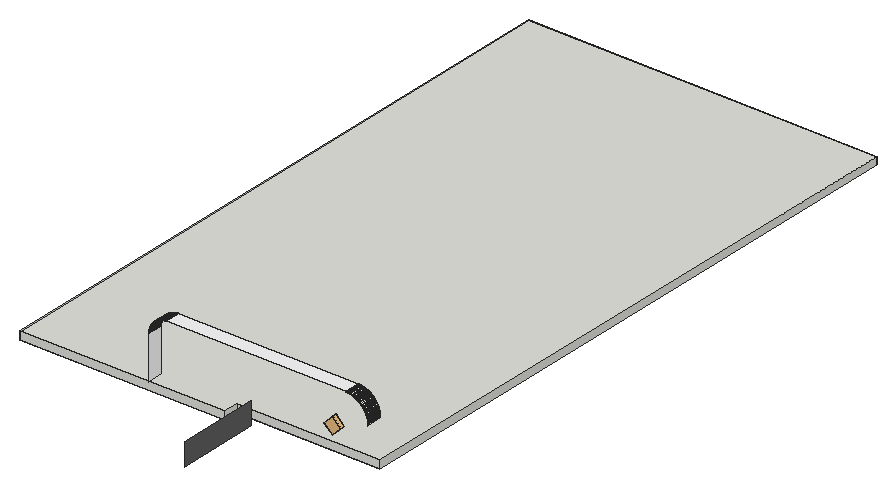
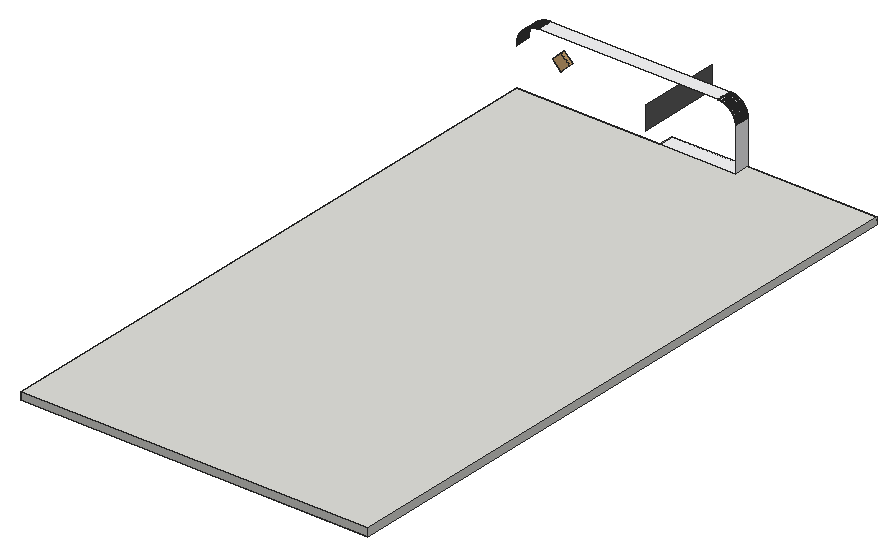
# SketchUp Ruby script. Lengths in inches.
U = 1.inch
M = Sketchup.active_model
def pt(a) = Geom::Point3d.new(a.map { |v| v * U })
def face(e, loops, mat)
  f = e.add_face(loops[0].map { |a| pt(a) })
  loops[1..].each { |l| e.add_face(l.map { |a| pt(a) }).erase! }
  f.material = f.back_material = mat if mat
  f
end
# faces: each face lists its corners as indices into pts; further lists are holes
def faces(e, pts, list, mat = nil) = list.each { |f| face(e, (f[0].is_a?(Array) ? f : [f]).map { |l| l.map { |i| pts[i] } }, mat) }
# xy, xz, yz: faces in a plane at the given z, y or x. An outline is a flat list of corners, or four numbers for a rectangle; further outlines are holes
def ring(l) = l.size == 4 ? [[l[0], l[1]], [l[2], l[1]], [l[2], l[3]], [l[0], l[3]]] : l.each_slice(2).to_a
def flat(e, list, mat, &to3) = list.each { |f| face(e, (f[0].is_a?(Array) ? f : [f]).map { |l| ring(l).map { |u, v| to3.(u, v) } }, mat) }
def xy(e, z, list, mat = nil) = flat(e, list, mat) { |x, y| [x, y, z] }
def xz(e, y, list, mat = nil) = flat(e, list, mat) { |x, z| [x, y, z] }
def yz(e, x, list, mat = nil) = flat(e, list, mat) { |y, z| [x, y, z] }
def lines(e, pts, list) = list.each { |a, b| e.add_line(pt(pts[a]), pt(pts[b])) }
# prism: a flat outline (further loops are holes) pulled along v
def prism(e, loops, v, mat = nil)
  f = face(e, loops, mat); d = Geom::Vector3d.new(v.map { |x| x * U })
  f.pushpull(f.normal.samedirection?(d) ? d.length : -d.length)
end
def box(e, o, s, mat = nil) = prism(e, [[o, [o[0] + s[0], o[1], o[2]], [o[0] + s[0], o[1] + s[1], o[2]], [o[0], o[1] + s[1], o[2]]]], [0, 0, s[2]], mat)
def at(x, y, z, deg = 0) = Geom::Transformation.translation(pt([x, y, z])) * Geom::Transformation.rotation(ORIGIN, Z_AXIS, deg.degrees)
def axes(o, x, y, z) = Geom::Transformation.new([*x, 0, *y, 0, *z, 0, *pt(o).to_a, 1])
def part(name) = M.definitions.add(name)
# library, detail: a bought-in or finely detailed component or shape, given as its bounding box
def library(name, o, s) = part(name).tap { |d| box(d.entities, o, s) }
def detail(e, o, s) = box(e.add_group.entities, o, s)
def put(e, d, t, mat = nil) = e.add_instance(d, t).tap { |i| i.material = mat if mat }
def group(e, t, mat = nil) = e.add_group.tap { |g| g.transformation = t; g.material = mat if mat }.entities
root = M.entities
M.materials.add("1421 AP 8232 ELEGANT GREY").color = [96, 96, 96]
M.materials.add("1448 AP 8253 RAVEN SONG").color = [0, 0, 0]
M.materials.add("[Quartz Light Grey]").color = [251, 251, 252]
c1 = library("Group\#22",[-1.75,-3,-1.85],[9.46,3.28,9.45])
xy(root,246,[[[36,271,198,271,198,283,312,283,312,775,36,775],[45,280,45,766,303,766,303,292,189,292,189,280]]])
xy(root,252,[[138,271,198,283]],"[Quartz Light Grey]")
xy(root,299.99,[[294.47,271,294.71,283]],"[Quartz Light Grey]")
xy(root,300,[[151.63,271,151.82,283],[151.82,271,152,283],[152,271,294,283],[294,271,294.24,283]],"[Quartz Light Grey]")
yz(root,138,[[271,252,283,286],[271,286,283,286.18],[271,286.18,283,286.37]],"[Quartz Light Grey]")
yz(root,219,[[205,249,271,267]],"1421 AP 8232 ELEGANT GREY")
yz(root,311.99,[[271,282.47,283,282.71]],"[Quartz Light Grey]")
yz(root,312,[[271,282,283,282.24]],"[Quartz Light Grey]")
p = [[311.99,271,282.47],[312,271,282.24],[312,283,282.24],[311.99,283,282.47],[311.98,271,282.94],[311.99,271,282.71],
  [311.99,283,282.71],[311.98,283,282.94],[311.96,271,283.18],[311.96,283,283.18],[311.94,271,283.41],[311.94,283,283.41],
  [311.92,271,283.65],[311.92,283,283.65],[311.9,271,283.88],[311.9,283,283.88],[311.875,271,284.12],[311.875,283,284.12],
  [311.85,271,284.35],[311.85,283,284.35],[311.8125,271,284.58],[311.8125,283,284.58],[311.78,271,284.82],[311.78,283,284.82],
  [311.74,271,285.05],[311.74,283,285.05],[311.7,271,285.28],[311.7,283,285.28],[311.65,271,285.51],[311.65,283,285.51],
  [311.61,271,285.74],[311.61,283,285.74],[311.56,271,285.97],[311.56,283,285.97],[311.5,271,286.2],[311.5,283,286.2],
  [311.45,271,286.43],[311.45,283,286.43],[138,271,286.37],[138.01,271,286.55],[138.01,283,286.55],[138,283,286.37],
  [311.39,271,286.66],[311.39,283,286.66],[138.02,271,286.73],[138.02,283,286.73],[138.03,271,286.92],[138.03,283,286.92],
  [311.32,271,286.89],[311.32,283,286.89],[138.04,271,287.1],[138.04,283,287.1],[311.26,271,287.11],[311.26,283,287.11],
  [138.06,271,287.28],[138.06,283,287.28],[311.19,271,287.34],[311.19,283,287.34],[138.08,271,287.46],[138.08,283,287.46],
  [311.12,271,287.5625],[311.12,283,287.5625],[138.1,271,287.65],[138.1,283,287.65],[138.12,271,287.83],[138.12,283,287.83],
  [311.04,271,287.79],[311.04,283,287.79],[138.14,271,288.01],[138.14,283,288.01],[310.97,271,288.01],[310.97,283,288.01],
  [138.17,271,288.19],[138.17,283,288.19],[310.89,271,288.23],[310.89,283,288.23],[138.2,271,288.37],[138.2,283,288.37],
  [310.8,271,288.45],[310.8,283,288.45],[138.23,271,288.55],[138.23,283,288.55],[310.72,271,288.67],[310.72,283,288.67],
  [138.27,271,288.73],[138.27,283,288.73],[138.31,271,288.91],[138.31,283,288.91],[310.63,271,288.89],[310.63,283,288.89],
  [138.35,271,289.09],[138.35,283,289.09],[310.54,271,289.11],[310.54,283,289.11],[138.39,271,289.27],[138.39,283,289.27],
  [310.44,271,289.32],[310.44,283,289.32],[138.43,271,289.45],[138.43,283,289.45],[310.35,271,289.54],[310.35,283,289.54],
  [138.48,271,289.625],[138.48,283,289.625],[310.25,271,289.75],[310.25,283,289.75],[138.53,271,289.8],[138.53,283,289.8],
  [310.14,271,289.96],[310.14,283,289.96],[138.58,271,289.98],[138.58,283,289.98],[138.63,271,290.15],[138.63,283,290.15],
  [310.04,271,290.17],[310.04,283,290.17],[138.69,271,290.33],[138.69,283,290.33],[309.93,271,290.38],[309.93,283,290.38],
  [138.74,271,290.5],[138.74,283,290.5],[309.82,271,290.59],[309.82,283,290.59],[138.8,271,290.67],[138.8,283,290.67],
  [309.7,271,290.8],[309.7,283,290.8],[138.87,271,290.85],[138.87,283,290.85],[138.93,271,291.02],[138.93,283,291.02],
  [309.59,271,291],[309.59,283,291],[139,271,291.1875],[139,283,291.1875],[309.47,271,291.2],[309.47,283,291.2],
  [139.07,271,291.36],[139.07,283,291.36],[309.35,271,291.4],[309.35,283,291.4],[139.14,271,291.53],[139.14,283,291.53],
  [309.22,271,291.61],[309.22,283,291.61],[139.21,271,291.69],[139.21,283,291.69],[309.1,271,291.8],[309.1,283,291.8],
  [139.29,271,291.86],[139.29,283,291.86],[308.97,271,292],[308.97,283,292],[139.36,271,292.03],[139.36,283,292.03],
  [139.44,271,292.19],[139.44,283,292.19],[308.83,271,292.2],[308.83,283,292.2],[139.53,271,292.36],[139.53,283,292.36],
  [308.7,271,292.39],[308.7,283,292.39],[139.61,271,292.52],[139.61,283,292.52],[308.5625,271,292.58],[308.5625,283,292.58],
  [139.7,271,292.68],[139.7,283,292.68],[308.42,271,292.77],[308.42,283,292.77],[139.79,271,292.84],[139.79,283,292.84],
  [139.875,271,293],[139.875,283,293],[308.28,271,292.96],[308.28,283,292.96],[139.97,271,293.16],[139.97,283,293.16],
  [308.14,271,293.14],[308.14,283,293.14],[307.99,271,293.33],[307.99,283,293.33],[140.0625,271,293.31],[140.0625,283,293.31],
  [140.16,271,293.47],[140.16,283,293.47],[307.84,271,293.51],[307.84,283,293.51],[140.26,271,293.625],[140.26,283,293.625],
  [307.6875,271,293.69],[307.6875,283,293.69],[140.36,271,293.78],[140.36,283,293.78],[307.53,271,293.87],[307.53,283,293.87],
  [140.46,271,293.93],[140.46,283,293.93],[140.57,271,294.08],[140.57,283,294.08],[307.375,271,294.04],[307.375,283,294.04],
  [307.22,271,294.22],[307.22,283,294.22],[140.67,271,294.23],[140.67,283,294.23],[140.78,271,294.375],[140.78,283,294.375],
  [307.06,271,294.39],[307.06,283,294.39],[140.89,271,294.52],[140.89,283,294.52],[306.89,271,294.56],[306.89,283,294.56],
  [141.01,271,294.67],[141.01,283,294.67],[306.73,271,294.73],[306.73,283,294.73],[141.12,271,294.81],[141.12,283,294.81],
  [306.56,271,294.89],[306.56,283,294.89],[141.24,271,294.95],[141.24,283,294.95],[306.39,271,295.06],[306.39,283,295.06],
  [141.35,271,295.09],[141.35,283,295.09],[141.47,271,295.23],[141.47,283,295.23],[306.22,271,295.22],[306.22,283,295.22],
  [141.6,271,295.37],[141.6,283,295.37],[306.04,271,295.375],[306.04,283,295.375],[141.72,271,295.5],[141.72,283,295.5],
  [305.87,271,295.53],[305.87,283,295.53],[141.84,271,295.64],[141.84,283,295.64],[305.69,271,295.6875],[305.69,283,295.6875],
  [141.97,271,295.77],[141.97,283,295.77],[305.51,271,295.84],[305.51,283,295.84],[142.1,271,295.9],[142.1,283,295.9],
  [305.33,271,295.99],[305.33,283,295.99],[142.23,271,296.03],[142.23,283,296.03],[142.36,271,296.16],[142.36,283,296.16],
  [305.14,271,296.14],[305.14,283,296.14],[304.96,271,296.28],[304.96,283,296.28],[142.5,271,296.28],[142.5,283,296.28],
  [142.63,271,296.4],[142.63,283,296.4],[304.77,271,296.42],[304.77,283,296.42],[142.77,271,296.53],[142.77,283,296.53],
  [304.58,271,296.5625],[304.58,283,296.5625],[142.91,271,296.65],[142.91,283,296.65],[143.05,271,296.76],[143.05,283,296.76],
  [304.39,271,296.7],[304.39,283,296.7],[304.2,271,296.83],[304.2,283,296.83],[143.19,271,296.88],[143.19,283,296.88],
  [304,271,296.97],[304,283,296.97],[143.33,271,296.99],[143.33,283,296.99],[143.48,271,297.11],[143.48,283,297.11],
  [303.8,271,297.1],[303.8,283,297.1],[143.625,271,297.22],[143.625,283,297.22],[303.61,271,297.22],[303.61,283,297.22],
  [143.77,271,297.33],[143.77,283,297.33],[303.4,271,297.35],[303.4,283,297.35],[143.92,271,297.43],[143.92,283,297.43],
  [303.2,271,297.47],[303.2,283,297.47],[144.07,271,297.54],[144.07,283,297.54],[144.22,271,297.64],[144.22,283,297.64],
  [303,271,297.59],[303,283,297.59],[144.375,271,297.74],[144.375,283,297.74],[302.8,271,297.7],[302.8,283,297.7],
  [144.53,271,297.84],[144.53,283,297.84],[302.59,271,297.82],[302.59,283,297.82],[144.69,271,297.9375],[144.69,283,297.9375],
  [302.38,271,297.93],[302.38,283,297.93],[144.84,271,298.03],[144.84,283,298.03],[302.17,271,298.04],[302.17,283,298.04],
  [145,271,298.125],[145,283,298.125],[301.96,271,298.14],[301.96,283,298.14],[145.16,271,298.21],[145.16,283,298.21],
  [301.75,271,298.25],[301.75,283,298.25],[145.32,271,298.3],[145.32,283,298.3],[301.54,271,298.35],[301.54,283,298.35],
  [145.48,271,298.39],[145.48,283,298.39],[301.32,271,298.44],[301.32,283,298.44],[145.64,271,298.47],[145.64,283,298.47],
  [301.11,271,298.54],[301.11,283,298.54],[145.81,271,298.56],[145.81,283,298.56],[300.89,271,298.63],[300.89,283,298.63],
  [145.97,271,298.64],[145.97,283,298.64],[146.14,271,298.71],[146.14,283,298.71],[300.67,271,298.72],[300.67,283,298.72],
  [146.31,271,298.79],[146.31,283,298.79],[300.45,271,298.8],[300.45,283,298.8],[146.47,271,298.86],[146.47,283,298.86],
  [300.23,271,298.89],[300.23,283,298.89],[146.64,271,298.93],[146.64,283,298.93],[146.8125,271,299],[146.8125,283,299],
  [300.01,271,298.97],[300.01,283,298.97],[146.98,271,299.07],[146.98,283,299.07],[299.5625,271,299.12],[299.79,271,299.04],
  [299.79,283,299.04],[299.5625,283,299.12],[147.15,271,299.13],[147.15,283,299.13],[147.33,271,299.2],[147.33,283,299.2],
  [299.34,271,299.19],[299.34,283,299.19],[147.5,271,299.26],[147.5,283,299.26],[299.11,271,299.26],[299.11,283,299.26],
  [147.67,271,299.31],[147.67,283,299.31],[147.85,271,299.37],[147.85,283,299.37],[298.66,271,299.39],[298.89,271,299.32],
  [298.89,283,299.32],[298.66,283,299.39],[148.02,271,299.42],[148.02,283,299.42],[148.2,271,299.47],[148.2,283,299.47],
  [298.2,271,299.5],[298.43,271,299.45],[298.43,283,299.45],[298.2,283,299.5],[148.375,271,299.52],[148.375,283,299.52],
  [148.55,271,299.57],[148.55,283,299.57],[297.97,271,299.56],[297.97,283,299.56],[148.73,271,299.61],[148.73,283,299.61],
  [148.91,271,299.65],[148.91,283,299.65],[297.51,271,299.65],[297.74,271,299.61],[297.74,283,299.61],[297.51,283,299.65],
  [149.09,271,299.69],[149.09,283,299.69],[149.27,271,299.73],[149.27,283,299.73],[149.45,271,299.77],[149.45,283,299.77],
  [296.82,271,299.78],[297.05,271,299.74],[297.05,283,299.74],[296.82,283,299.78],[297.28,271,299.7],[297.28,283,299.7],
  [149.63,271,299.8],[149.63,283,299.8],[149.81,271,299.83],[149.81,283,299.83],[149.99,271,299.86],[149.99,283,299.86],
  [296.12,271,299.875],[296.35,271,299.85],[296.35,283,299.85],[296.12,283,299.875],[296.58,271,299.8125],[296.58,283,299.8125],
  [150.17,271,299.88],[150.17,283,299.88],[150.35,271,299.9],[150.35,283,299.9],[150.54,271,299.92],[150.54,283,299.92],
  [150.72,271,299.94],[150.72,283,299.94],[150.9,271,299.96],[150.9,283,299.96],[295.18,271,299.96],[295.41,271,299.94],
  [295.41,283,299.94],[295.18,283,299.96],[295.65,271,299.92],[295.65,283,299.92],[295.88,271,299.9],[295.88,283,299.9],
  [151.08,271,299.97],[151.08,283,299.97],[151.27,271,299.98],[151.27,283,299.98],[151.45,271,299.99],[151.45,283,299.99],
  [151.63,271,300],[151.63,283,300],[294.24,271,300],[294.47,271,299.99],[294.47,283,299.99],[294.24,283,300],
  [294.71,271,299.99],[294.94,271,299.98],[294.94,283,299.98],[294.71,283,299.99]]
faces(root,p,[[0,1,2,3],[4,5,6,7],[8,4,7,9],[10,8,9,11],[12,10,11,13],[14,12,13,15],[16,14,15,17],[18,16,17,19],
  [20,18,19,21],[22,20,21,23],[24,22,23,25],[26,24,25,27],[28,26,27,29],[30,28,29,31],[32,30,31,33],[34,32,33,35],
  [36,34,35,37],[38,39,40,41],[42,36,37,43],[39,44,45,40],[44,46,47,45],[48,42,43,49],[46,50,51,47],[52,48,49,53],
  [50,54,55,51],[56,52,53,57],[54,58,59,55],[60,56,57,61],[58,62,63,59],[62,64,65,63],[66,60,61,67],[64,68,69,65],
  [70,66,67,71],[68,72,73,69],[74,70,71,75],[72,76,77,73],[78,74,75,79],[76,80,81,77],[82,78,79,83],[80,84,85,81],
  [84,86,87,85],[88,82,83,89],[86,90,91,87],[92,88,89,93],[90,94,95,91],[96,92,93,97],[94,98,99,95],[100,96,97,101],
  [98,102,103,99],[104,100,101,105],[102,106,107,103],[108,104,105,109],[106,110,111,107],[110,112,113,111],[114,108,109,115],[112,116,117,113],
  [118,114,115,119],[116,120,121,117],[122,118,119,123],[120,124,125,121],[126,122,123,127],[124,128,129,125],[128,130,131,129],[132,126,127,133],
  [130,134,135,131],[136,132,133,137],[134,138,139,135],[140,136,137,141],[138,142,143,139],[144,140,141,145],[142,146,147,143],[148,144,145,149],
  [146,150,151,147],[152,148,149,153],[150,154,155,151],[154,156,157,155],[158,152,153,159],[156,160,161,157],[162,158,159,163],[160,164,165,161],
  [166,162,163,167],[164,168,169,165],[170,166,167,171],[168,172,173,169],[172,174,175,173],[176,170,171,177],[174,178,179,175],[180,176,177,181],
  [182,180,181,183],[178,184,185,179],[184,186,187,185],[188,182,183,189],[186,190,191,187],[192,188,189,193],[190,194,195,191],[196,192,193,197],
  [194,198,199,195],[198,200,201,199],[202,196,197,203],[204,202,203,205],[200,206,207,201],[206,208,209,207],[210,204,205,211],[208,212,213,209],
  [214,210,211,215],[212,216,217,213],[218,214,215,219],[216,220,221,217],[222,218,219,223],[220,224,225,221],[226,222,223,227],[224,228,229,225],
  [228,230,231,229],[232,226,227,233],[230,234,235,231],[236,232,233,237],[234,238,239,235],[240,236,237,241],[238,242,243,239],[244,240,241,245],
  [242,246,247,243],[248,244,245,249],[246,250,251,247],[252,248,249,253],[250,254,255,251],[254,256,257,255],[258,252,253,259],[260,258,259,261],
  [256,262,263,257],[262,264,265,263],[266,260,261,267],[264,268,269,265],[270,266,267,271],[268,272,273,269],[272,274,275,273],[276,270,271,277],
  [278,276,277,279],[274,280,281,275],[282,278,279,283],[280,284,285,281],[284,286,287,285],[288,282,283,289],[286,290,291,287],[292,288,289,293],
  [290,294,295,291],[296,292,293,297],[294,298,299,295],[300,296,297,301],[298,302,303,299],[302,304,305,303],[306,300,301,307],[304,308,309,305],
  [310,306,307,311],[308,312,313,309],[314,310,311,315],[312,316,317,313],[318,314,315,319],[316,320,321,317],[322,318,319,323],[320,324,325,321],
  [326,322,323,327],[324,328,329,325],[330,326,327,331],[328,332,333,329],[334,330,331,335],[332,336,337,333],[338,334,335,339],[336,340,341,337],
  [342,338,339,343],[340,344,345,341],[346,342,343,347],[344,348,349,345],[348,350,351,349],[352,346,347,353],[350,354,355,351],[356,352,353,357],
  [354,358,359,355],[360,356,357,361],[358,362,363,359],[362,364,365,363],[366,360,361,367],[364,368,369,365],[370,371,372,373],[371,366,367,372],
  [368,374,375,369],[374,376,377,375],[378,370,373,379],[376,380,381,377],[382,378,379,383],[380,384,385,381],[384,386,387,385],[388,389,390,391],
  [389,382,383,390],[386,392,393,387],[392,394,395,393],[396,397,398,399],[397,388,391,398],[394,400,401,395],[400,402,403,401],[404,396,399,405],
  [402,406,407,403],[406,408,409,407],[410,411,412,413],[411,404,405,412],[408,414,415,409],[414,416,417,415],[416,418,419,417],[420,421,422,423],
  [421,424,425,422],[424,410,413,425],[418,426,427,419],[426,428,429,427],[428,430,431,429],[432,433,434,435],[433,436,437,434],[436,420,423,437],
  [430,438,439,431],[438,440,441,439],[440,442,443,441],[442,444,445,443],[444,446,447,445],[448,449,450,451],[449,452,453,450],[452,454,455,453],
  [454,432,435,455],[446,456,457,447],[456,458,459,457],[458,460,461,459],[460,462,463,461],[464,465,466,467],[468,469,470,471],[469,448,451,470]],"[Quartz Light Grey]")
put(root,c1,axes([285.96,271,269.85],[0.70711,0,0.70711],[0,1,0],[-0.70711,0,0.70711]),"1448 AP 8253 RAVEN SONG")
g1 = group(root,at(36,271,246))
prism(g1,[[[276,504,0],[276,12,0],[162,12,0],[162,0,0],[0,0,0],[0,504,0]]],[0,0,6])
